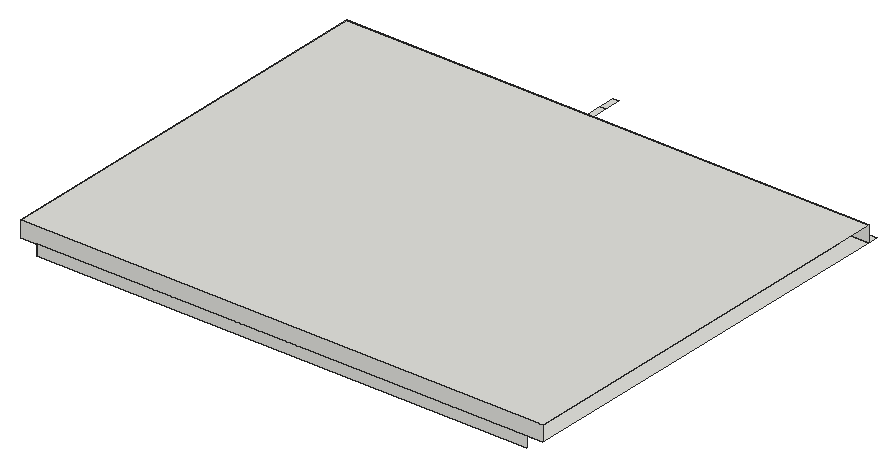
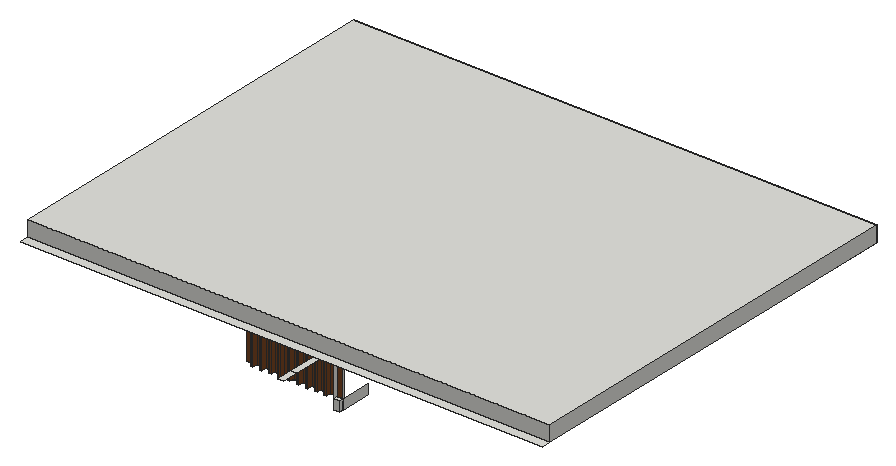
# SketchUp Ruby script. Lengths in inches.
U = 1.inch
M = Sketchup.active_model
def pt(a) = Geom::Point3d.new(a.map { |v| v * U })
def face(e, loops, mat)
  f = e.add_face(loops[0].map { |a| pt(a) })
  loops[1..].each { |l| e.add_face(l.map { |a| pt(a) }).erase! }
  f.material = f.back_material = mat if mat
  f
end
# faces: each face lists its corners as indices into pts; further lists are holes
def faces(e, pts, list, mat = nil) = list.each { |f| face(e, (f[0].is_a?(Array) ? f : [f]).map { |l| l.map { |i| pts[i] } }, mat) }
# xy, xz, yz: faces in a plane at the given z, y or x. An outline is a flat list of corners, or four numbers for a rectangle; further outlines are holes
def ring(l) = l.size == 4 ? [[l[0], l[1]], [l[2], l[1]], [l[2], l[3]], [l[0], l[3]]] : l.each_slice(2).to_a
def flat(e, list, mat, &to3) = list.each { |f| face(e, (f[0].is_a?(Array) ? f : [f]).map { |l| ring(l).map { |u, v| to3.(u, v) } }, mat) }
def xy(e, z, list, mat = nil) = flat(e, list, mat) { |x, y| [x, y, z] }
def xz(e, y, list, mat = nil) = flat(e, list, mat) { |x, z| [x, y, z] }
def yz(e, x, list, mat = nil) = flat(e, list, mat) { |y, z| [x, y, z] }
def lines(e, pts, list) = list.each { |a, b| e.add_line(pt(pts[a]), pt(pts[b])) }
# prism: a flat outline (further loops are holes) pulled along v
def prism(e, loops, v, mat = nil)
  f = face(e, loops, mat); d = Geom::Vector3d.new(v.map { |x| x * U })
  f.pushpull(f.normal.samedirection?(d) ? d.length : -d.length)
end
def box(e, o, s, mat = nil) = prism(e, [[o, [o[0] + s[0], o[1], o[2]], [o[0] + s[0], o[1] + s[1], o[2]], [o[0], o[1] + s[1], o[2]]]], [0, 0, s[2]], mat)
def at(x, y, z, deg = 0) = Geom::Transformation.translation(pt([x, y, z])) * Geom::Transformation.rotation(ORIGIN, Z_AXIS, deg.degrees)
def axes(o, x, y, z) = Geom::Transformation.new([*x, 0, *y, 0, *z, 0, *pt(o).to_a, 1])
def part(name) = M.definitions.add(name)
# library, detail: a bought-in or finely detailed component or shape, given as its bounding box
def library(name, o, s) = part(name).tap { |d| box(d.entities, o, s) }
def detail(e, o, s) = box(e.add_group.entities, o, s)
def put(e, d, t, mat = nil) = e.add_instance(d, t).tap { |i| i.material = mat if mat }
def group(e, t, mat = nil) = e.add_group.tap { |g| g.transformation = t; g.material = mat if mat }.entities
root = M.entities
M.materials.add("[Color C01]").color = [255, 229, 204]
M.materials.add("[Wood Veneer 01]").color = [120, 70, 37]
c1 = library("Avation+Styled+Ceiling+Fan_JSB",[-19.77,-29.63,-13.8125],[51.59,58.16,13.8125])
xy(root,101.64,[[84.82,147.02,87.24,148.71]])
xy(root,102.39,[[108.65,138.59,108.1,138.66,107.59,138.87,107.15,139.21,106.81,139.65,106.6,140.16,106.52,140.71,106.6,141.26,106.81,141.77,107.15,142.21,107.59,142.55,108.1,142.76,108.65,142.84,109.2,142.76,109.71,142.55,110.15,142.21,110.49,141.77,110.7,141.26,110.77,140.71,110.7,140.16,110.49,139.65,110.15,139.21,109.71,138.87,109.2,138.66]])
xy(root,105.33,[[84.82,147.02,87.24,148.71]])
xy(root,119.8125,[[87.24,147.02,89.8,148.71],[90.74,147.02,93.3,148.71],[94.24,147.02,96.8,148.71],[97.74,147.02,100.3,148.71],[101.24,147.02,103.8,148.71],
  [104.74,147.02,107.3,148.71],[108.24,147.02,110.8,148.71],[111.74,147.02,114.3,148.71],[115.24,147.02,117.8,148.71],[6.1,147.26,84.82,148.71]])
xy(root,119.8125,[[23.52,17.41,26.22,131.3],[26.64,17.41,29.35,131.3],[[29.77,17.41,32.47,131.3],[31.02,80.58,31.35,80.59,31.66,80.68,31.9375,80.85,32.16,81.08,32.32,81.37,32.4,81.6875,32.39,82.01,32.3,82.33,32.13,82.61,31.89,82.83,31.61,82.99,31.29,83.06,30.97,83.06,30.65,82.97,30.375,82.8,30.15,82.5625,29.99,82.27,29.91,81.96,29.92,81.63,30.01,81.32,30.18,81.04,30.42,80.8125,30.7,80.66]],[32.89,17.41,35.6,131.3],[36.02,17.41,38.72,131.3],
  [39.14,17.41,41.85,131.3]],"[Wood Veneer 01]")
xy(root,120.5,[[18.23,8.31,17.27,8.41,16.37,8.74,15.59,9.3,14.98,10.04,14.58,10.92,14.42,11.87,14.51,12.83,14.85,13.73,15.4,14.51,16.15,15.125,17.02,15.53,17.97,15.69,18.93,15.59,19.83,15.26,20.62,14.7,21.23,13.96,21.63,13.08,21.79,12.13,21.7,11.17,21.36,10.27,20.8,9.49,20.06,8.875,19.18,8.47],[99.22,8.5,98.3125,8.62,97.47,8.97,96.74,9.53,96.1875,10.25,95.84,11.09,95.72,12,95.84,12.91,96.1875,13.75,96.74,14.47,97.47,15.03,98.3125,15.38,99.22,15.5,100.125,15.38,100.97,15.03,101.69,14.47,102.25,13.75,102.6,12.91,102.72,12,102.6,11.09,102.25,10.25,101.69,9.53,100.97,8.97,100.125,8.62],[17.86,70.55,16.89,70.74,15.99,71.18,15.24,71.83,14.6875,72.66,14.36,73.6,14.3,74.6,14.49,75.57,14.93,76.47,15.58,77.22,16.41,77.77,17.35,78.09,18.34,78.16,19.32,77.97,20.21,77.53,20.96,76.875,21.52,76.05,21.84,75.11,21.91,74.12,21.72,73.14,21.28,72.24,20.625,71.49,19.8,70.94,18.86,70.62],[18.1,132.84,17.1,132.97,16.16,133.35,15.36,133.97,14.75,134.77,14.36,135.71,14.23,136.71,14.36,137.71,14.75,138.65,15.36,139.45,16.16,140.07,17.1,140.45,18.1,140.59,19.11,140.45,20.04,140.07,20.84,139.45,21.46,138.65,21.85,137.71,21.98,136.71,21.85,135.71,21.46,134.77,20.84,133.97,20.04,133.35,19.11,132.97],[99.22,133.4,98.36,133.51,97.5625,133.84,96.875,134.37,96.35,135.05,96.02,135.85,95.91,136.71,96.02,137.57,96.35,138.37,96.875,139.05,97.5625,139.58,98.36,139.91,99.22,140.02,100.08,139.91,100.875,139.58,101.5625,139.05,102.09,138.37,102.42,137.57,102.53,136.71,102.42,135.85,102.09,135.05,101.5625,134.37,100.875,133.84,100.08,133.51]])
xy(root,121.5,[[31.02,80.58,30.7,80.66,30.42,80.8125,30.18,81.04,30.01,81.32,29.92,81.63,29.91,81.96,29.99,82.27,30.15,82.5625,30.375,82.8,30.65,82.97,30.97,83.06,31.29,83.06,31.61,82.99,31.89,82.83,32.13,82.61,32.3,82.33,32.39,82.01,32.4,81.6875,32.32,81.37,32.16,81.08,31.9375,80.85,31.66,80.68,31.35,80.59]])
xy(root,123.25,[[26.22,17.41,26.64,131.3],[29.35,17.41,29.77,131.3],[32.47,17.41,32.89,131.3],[35.6,17.41,36.02,131.3],[38.72,17.41,39.14,131.3]])
xy(root,123.25,[[41.85,17.41,157.97,131.3]],"[Color C01]")
xy(root,123.71,[[84.82,147.02,87.07,147.26],[84.82,147.26,87.07,148.71],[84.82,148.71,87.07,154.8125],[84.82,154.8125,87.07,169.1875],[84.82,169.1875,87.07,175.3125]])
xy(root,123.75,[[0,0,0,154.8125,198.4375,154.8125,198.4375,0,192.34,0,192.34,148.71,6.1,148.71,6.1,0],[6.1,0,192.34,148.71],[0,154.8125,198.4375,158.375]])
xy(root,129.75,[[0,0,198.4375,154.8125]])
xz(root,0,[[6.1,119.8125,192.34,123.75],[0,123.75,198.4375,129.75]])
xz(root,17.41,[[26.22,119.8125,26.64,123.25],[29.35,119.8125,29.77,123.25],[32.47,119.8125,32.89,123.25],[35.6,119.8125,36.02,123.25],[38.72,119.8125,39.14,123.25],
  [41.85,119.8125,157.97,123.25]])
xz(root,83.06,[[30.97,119.8125,31.29,121.5]])
xz(root,131.3,[[26.22,119.8125,26.64,123.25],[29.35,119.8125,29.77,123.25],[32.47,119.8125,32.89,123.25],[35.6,119.8125,36.02,123.25],[38.72,119.8125,39.14,123.25]])
xz(root,131.3,[[41.85,119.8125,157.97,123.25]],"[Color C01]")
xz(root,147.02,[[84.82,101.64,87.07,105.33]])
xz(root,147.02,[[84.82,105.33,87.07,123.71],[87.24,105.33,89.8,119.8125],[90.74,105.33,93.3,119.8125],[94.24,105.33,96.8,119.8125],[97.74,105.33,100.3,119.8125],
  [101.24,105.33,103.8,119.8125],[104.74,105.33,107.3,119.8125],[108.24,105.33,110.8,119.8125],[111.74,105.33,114.3,119.8125],[115.24,105.33,117.8,119.8125],
  [118.74,105.33,121.3,119.8125]],"[Wood Veneer 01]")
xz(root,148.71,[[84.82,101.64,87.07,105.33],[87.07,101.64,87.24,105.33],[84.82,119.8125,87.07,123.71]])
xz(root,148.71,[[87.07,105.33,87.24,119.8125],[89.8,105.33,90.74,119.8125],[93.3,105.33,94.24,119.8125],[96.8,105.33,97.74,119.8125],[100.3,105.33,101.24,119.8125],
  [103.8,105.33,104.74,119.8125],[107.3,105.33,108.24,119.8125],[110.8,105.33,111.74,119.8125],[114.3,105.33,115.24,119.8125],[117.8,105.33,118.74,119.8125]],"[Wood Veneer 01]")
xz(root,154.8125,[[0,123.75,198.4375,129.75]])
yz(root,0,[[0,123.75,154.8125,129.75]])
yz(root,6.1,[[0,119.8125,148.71,123.75]])
yz(root,26.22,[[17.41,119.8125,131.3,123.25]],"[Wood Veneer 01]")
yz(root,26.64,[[17.41,119.8125,131.3,123.25]])
yz(root,29.35,[[17.41,119.8125,131.3,123.25]],"[Wood Veneer 01]")
yz(root,29.77,[[17.41,119.8125,131.3,123.25]])
yz(root,32.47,[[17.41,119.8125,131.3,123.25]],"[Wood Veneer 01]")
yz(root,32.89,[[17.41,119.8125,131.3,123.25]])
yz(root,35.6,[[17.41,119.8125,131.3,123.25]],"[Wood Veneer 01]")
yz(root,36.02,[[17.41,119.8125,131.3,123.25]],"[Wood Veneer 01]")
yz(root,38.72,[[17.41,119.8125,131.3,123.25]],"[Wood Veneer 01]")
yz(root,39.14,[[17.41,119.8125,131.3,123.25]],"[Wood Veneer 01]")
yz(root,41.85,[[17.41,119.8125,131.3,123.25]],"[Wood Veneer 01]")
yz(root,84.82,[[135.46,101.64,147.02,105.33],[147.02,101.64,147.26,105.33],[147.26,101.64,148.71,105.33],[147.02,105.33,147.26,123.71],[147.26,119.8125,148.71,123.71]])
yz(root,87.24,[[147.02,105.33,148.71,119.8125]])
yz(root,89.8,[[147.02,105.33,148.71,119.8125]],"[Wood Veneer 01]")
yz(root,90.74,[[147.02,105.33,148.71,119.8125]])
yz(root,93.3,[[147.02,105.33,148.71,119.8125]],"[Wood Veneer 01]")
yz(root,94.24,[[147.02,105.33,148.71,119.8125]])
yz(root,96.8,[[147.02,105.33,148.71,119.8125]],"[Wood Veneer 01]")
yz(root,97.74,[[147.02,105.33,148.71,119.8125]])
yz(root,100.3,[[147.02,105.33,148.71,119.8125]],"[Wood Veneer 01]")
yz(root,101.24,[[147.02,105.33,148.71,119.8125]])
yz(root,103.8,[[147.02,105.33,148.71,119.8125]],"[Wood Veneer 01]")
yz(root,104.74,[[147.02,105.33,148.71,119.8125]])
yz(root,107.3,[[147.02,105.33,148.71,119.8125]],"[Wood Veneer 01]")
yz(root,108.24,[[147.02,105.33,148.71,119.8125]])
yz(root,110.8,[[147.02,105.33,148.71,119.8125]],"[Wood Veneer 01]")
yz(root,111.74,[[147.02,105.33,148.71,119.8125]])
yz(root,114.3,[[147.02,105.33,148.71,119.8125]],"[Wood Veneer 01]")
yz(root,115.24,[[147.02,105.33,148.71,119.8125]])
yz(root,117.8,[[147.02,105.33,148.71,119.8125]],"[Wood Veneer 01]")
yz(root,118.74,[[147.02,105.33,148.71,119.8125]])
p = [[108.65,138.59,101.64],[108.1,138.66,101.64],[108.1,138.66,102.39],[108.65,138.59,102.39],[109.2,138.66,101.64],[109.2,138.66,102.39],
  [107.59,138.87,101.64],[107.59,138.87,102.39],[109.71,138.87,101.64],[109.71,138.87,102.39],[107.15,139.21,101.64],[107.15,139.21,102.39],
  [110.15,139.21,101.64],[110.15,139.21,102.39],[106.81,139.65,101.64],[106.81,139.65,102.39],[110.49,139.65,101.64],[110.49,139.65,102.39],
  [106.6,140.16,101.64],[106.6,140.16,102.39],[110.7,140.16,101.64],[110.7,140.16,102.39],[106.52,140.71,101.64],[106.52,140.71,102.39],
  [110.77,140.71,101.64],[110.77,140.71,102.39],[106.6,141.26,101.64],[106.6,141.26,102.39],[110.7,141.26,101.64],[110.7,141.26,102.39],
  [106.81,141.77,101.64],[106.81,141.77,102.39],[110.49,141.77,101.64],[110.49,141.77,102.39],[107.15,142.21,101.64],[107.15,142.21,102.39],
  [110.15,142.21,101.64],[110.15,142.21,102.39],[107.59,142.55,101.64],[107.59,142.55,102.39],[109.71,142.55,101.64],[109.71,142.55,102.39],
  [108.1,142.76,101.64],[108.1,142.76,102.39],[109.2,142.76,101.64],[109.2,142.76,102.39],[108.65,142.84,101.64],[108.65,142.84,102.39],
  [18.23,8.31,119.8125],[17.27,8.41,119.8125],[17.27,8.41,120.5],[18.23,8.31,120.5],[19.18,8.47,119.8125],[19.18,8.47,120.5],
  [16.37,8.74,119.8125],[16.37,8.74,120.5],[20.06,8.875,119.8125],[20.06,8.875,120.5],[99.22,8.5,119.8125],[98.3125,8.62,119.8125],
  [98.3125,8.62,120.5],[99.22,8.5,120.5],[100.125,8.62,119.8125],[100.125,8.62,120.5],[97.47,8.97,119.8125],[97.47,8.97,120.5],
  [100.97,8.97,119.8125],[100.97,8.97,120.5],[15.59,9.3,119.8125],[15.59,9.3,120.5],[20.8,9.49,119.8125],[20.8,9.49,120.5],
  [96.74,9.53,119.8125],[96.74,9.53,120.5],[101.69,9.53,119.8125],[101.69,9.53,120.5],[14.98,10.04,119.8125],[14.98,10.04,120.5],
  [21.36,10.27,119.8125],[21.36,10.27,120.5],[96.1875,10.25,119.8125],[96.1875,10.25,120.5],[102.25,10.25,119.8125],[102.25,10.25,120.5],
  [14.58,10.92,119.8125],[14.58,10.92,120.5],[95.84,11.09,119.8125],[95.84,11.09,120.5],[102.6,11.09,119.8125],[102.6,11.09,120.5],
  [21.7,11.17,119.8125],[21.7,11.17,120.5],[14.42,11.87,119.8125],[14.42,11.87,120.5],[95.72,12,119.8125],[95.72,12,120.5],
  [102.72,12,119.8125],[102.72,12,120.5],[21.79,12.13,119.8125],[21.79,12.13,120.5],[14.51,12.83,119.8125],[14.51,12.83,120.5],
  [95.84,12.91,119.8125],[95.84,12.91,120.5],[102.6,12.91,119.8125],[102.6,12.91,120.5],[21.63,13.08,119.8125],[21.63,13.08,120.5],
  [14.85,13.73,119.8125],[14.85,13.73,120.5],[96.1875,13.75,119.8125],[96.1875,13.75,120.5],[102.25,13.75,119.8125],[102.25,13.75,120.5],
  [21.23,13.96,119.8125],[21.23,13.96,120.5],[15.4,14.51,119.8125],[15.4,14.51,120.5],[96.74,14.47,119.8125],[96.74,14.47,120.5],
  [101.69,14.47,119.8125],[101.69,14.47,120.5],[20.62,14.7,119.8125],[20.62,14.7,120.5],[16.15,15.125,119.8125],[16.15,15.125,120.5],
  [97.47,15.03,119.8125],[97.47,15.03,120.5],[100.97,15.03,119.8125],[100.97,15.03,120.5],[19.83,15.26,119.8125],[19.83,15.26,120.5],
  [98.3125,15.38,119.8125],[98.3125,15.38,120.5],[100.125,15.38,119.8125],[100.125,15.38,120.5],[17.02,15.53,119.8125],[17.02,15.53,120.5],
  [18.93,15.59,119.8125],[18.93,15.59,120.5],[99.22,15.5,119.8125],[99.22,15.5,120.5],[17.97,15.69,119.8125],[17.97,15.69,120.5],
  [17.86,70.55,119.8125],[16.89,70.74,119.8125],[16.89,70.74,120.5],[17.86,70.55,120.5],[18.86,70.62,119.8125],[18.86,70.62,120.5],
  [19.8,70.94,119.8125],[19.8,70.94,120.5],[15.99,71.18,119.8125],[15.99,71.18,120.5],[20.625,71.49,119.8125],[20.625,71.49,120.5],
  [15.24,71.83,119.8125],[15.24,71.83,120.5],[21.28,72.24,119.8125],[21.28,72.24,120.5],[14.6875,72.66,119.8125],[14.6875,72.66,120.5],
  [21.72,73.14,119.8125],[21.72,73.14,120.5],[14.36,73.6,119.8125],[14.36,73.6,120.5],[21.91,74.12,119.8125],[21.91,74.12,120.5],
  [14.3,74.6,119.8125],[14.3,74.6,120.5],[21.84,75.11,119.8125],[21.84,75.11,120.5],[14.49,75.57,119.8125],[14.49,75.57,120.5],
  [21.52,76.05,119.8125],[21.52,76.05,120.5],[14.93,76.47,119.8125],[14.93,76.47,120.5],[20.96,76.875,119.8125],[20.96,76.875,120.5],
  [15.58,77.22,119.8125],[15.58,77.22,120.5],[20.21,77.53,119.8125],[20.21,77.53,120.5],[16.41,77.77,119.8125],[16.41,77.77,120.5],
  [19.32,77.97,119.8125],[19.32,77.97,120.5],[17.35,78.09,119.8125],[17.35,78.09,120.5],[18.34,78.16,119.8125],[18.34,78.16,120.5],
  [31.02,80.58,119.8125],[30.7,80.66,119.8125],[30.7,80.66,121.5],[31.02,80.58,121.5],[31.35,80.59,119.8125],[31.35,80.59,121.5],
  [31.66,80.68,119.8125],[31.66,80.68,121.5],[30.42,80.8125,119.8125],[30.42,80.8125,121.5],[31.9375,80.85,119.8125],[31.9375,80.85,121.5],
  [30.18,81.04,119.8125],[30.18,81.04,121.5],[32.16,81.08,119.8125],[32.16,81.08,121.5],[30.01,81.32,119.8125],[30.01,81.32,121.5],
  [32.32,81.37,119.8125],[32.32,81.37,121.5],[29.92,81.63,119.8125],[29.92,81.63,121.5],[32.4,81.6875,119.8125],[32.4,81.6875,121.5],
  [29.91,81.96,119.8125],[29.91,81.96,121.5],[32.39,82.01,119.8125],[32.39,82.01,121.5],[29.99,82.27,119.8125],[29.99,82.27,121.5],
  [32.3,82.33,119.8125],[32.3,82.33,121.5],[30.15,82.5625,119.8125],[30.15,82.5625,121.5],[32.13,82.61,119.8125],[32.13,82.61,121.5],
  [30.375,82.8,119.8125],[30.375,82.8,121.5],[31.89,82.83,119.8125],[31.89,82.83,121.5],[30.65,82.97,119.8125],[30.65,82.97,121.5],
  [31.61,82.99,119.8125],[31.61,82.99,121.5],[30.97,83.06,119.8125],[30.97,83.06,121.5],[31.29,83.06,119.8125],[31.29,83.06,121.5],
  [18.1,132.84,119.8125],[17.1,132.97,119.8125],[17.1,132.97,120.5],[18.1,132.84,120.5],[19.11,132.97,119.8125],[19.11,132.97,120.5],
  [16.16,133.35,119.8125],[16.16,133.35,120.5],[20.04,133.35,119.8125],[20.04,133.35,120.5],[15.36,133.97,119.8125],[15.36,133.97,120.5],
  [20.84,133.97,119.8125],[20.84,133.97,120.5],[99.22,133.4,119.8125],[98.36,133.51,119.8125],[98.36,133.51,120.5],[99.22,133.4,120.5],
  [100.08,133.51,119.8125],[100.08,133.51,120.5],[97.5625,133.84,119.8125],[97.5625,133.84,120.5],[100.875,133.84,119.8125],[100.875,133.84,120.5],
  [96.875,134.37,119.8125],[96.875,134.37,120.5],[101.5625,134.37,119.8125],[101.5625,134.37,120.5],[14.75,134.77,119.8125],[14.75,134.77,120.5],
  [21.46,134.77,119.8125],[21.46,134.77,120.5],[96.35,135.05,119.8125],[96.35,135.05,120.5],[102.09,135.05,119.8125],[102.09,135.05,120.5],
  [14.36,135.71,119.8125],[14.36,135.71,120.5],[21.85,135.71,119.8125],[21.85,135.71,120.5],[96.02,135.85,119.8125],[96.02,135.85,120.5],
  [102.42,135.85,119.8125],[102.42,135.85,120.5],[14.23,136.71,119.8125],[14.23,136.71,120.5],[21.98,136.71,119.8125],[21.98,136.71,120.5],
  [95.91,136.71,119.8125],[95.91,136.71,120.5],[102.53,136.71,119.8125],[102.53,136.71,120.5],[14.36,137.71,119.8125],[14.36,137.71,120.5],
  [21.85,137.71,119.8125],[21.85,137.71,120.5],[96.02,137.57,119.8125],[96.02,137.57,120.5],[102.42,137.57,119.8125],[102.42,137.57,120.5],
  [96.35,138.37,119.8125],[96.35,138.37,120.5],[102.09,138.37,119.8125],[102.09,138.37,120.5],[14.75,138.65,119.8125],[14.75,138.65,120.5],
  [21.46,138.65,119.8125],[21.46,138.65,120.5],[96.875,139.05,119.8125],[96.875,139.05,120.5],[101.5625,139.05,119.8125],[101.5625,139.05,120.5],
  [15.36,139.45,119.8125],[15.36,139.45,120.5],[20.84,139.45,119.8125],[20.84,139.45,120.5],[97.5625,139.58,119.8125],[97.5625,139.58,120.5],
  [100.875,139.58,119.8125],[100.875,139.58,120.5],[16.16,140.07,119.8125],[16.16,140.07,120.5],[20.04,140.07,119.8125],[20.04,140.07,120.5],
  [98.36,139.91,119.8125],[98.36,139.91,120.5],[100.08,139.91,119.8125],[100.08,139.91,120.5],[99.22,140.02,119.8125],[99.22,140.02,120.5],
  [17.1,140.45,119.8125],[17.1,140.45,120.5],[19.11,140.45,119.8125],[19.11,140.45,120.5],[18.1,140.59,119.8125],[18.1,140.59,120.5]]
faces(root,p,[[0,1,2,3],[4,0,3,5],[1,6,7,2],[8,4,5,9],[6,10,11,7],[12,8,9,13],[10,14,15,11],[16,12,13,17],
  [14,18,19,15],[20,16,17,21],[18,22,23,19],[24,20,21,25],[22,26,27,23],[28,24,25,29],[26,30,31,27],[32,28,29,33],
  [30,34,35,31],[36,32,33,37],[34,38,39,35],[40,36,37,41],[38,42,43,39],[44,40,41,45],[42,46,47,43],[46,44,45,47],
  [48,49,50,51],[52,48,51,53],[49,54,55,50],[56,52,53,57],[58,59,60,61],[62,58,61,63],[59,64,65,60],[66,62,63,67],
  [54,68,69,55],[70,56,57,71],[64,72,73,65],[74,66,67,75],[68,76,77,69],[78,70,71,79],[72,80,81,73],[82,74,75,83],
  [76,84,85,77],[80,86,87,81],[88,82,83,89],[90,78,79,91],[84,92,93,85],[86,94,95,87],[96,88,89,97],[98,90,91,99],
  [92,100,101,93],[94,102,103,95],[104,96,97,105],[106,98,99,107],[100,108,109,101],[102,110,111,103],[112,104,105,113],[114,106,107,115],
  [108,116,117,109],[110,118,119,111],[120,112,113,121],[122,114,115,123],[116,124,125,117],[118,126,127,119],[128,120,121,129],[130,122,123,131],
  [126,132,133,127],[134,128,129,135],[124,136,137,125],[138,130,131,139],[132,140,141,133],[140,134,135,141],[136,142,143,137],[142,138,139,143],
  [144,145,146,147],[148,144,147,149],[150,148,149,151],[145,152,153,146],[154,150,151,155],[152,156,157,153],[158,154,155,159],[156,160,161,157],
  [162,158,159,163],[160,164,165,161],[166,162,163,167],[164,168,169,165],[170,166,167,171],[168,172,173,169],[174,170,171,175],[172,176,177,173],
  [178,174,175,179],[176,180,181,177],[182,178,179,183],[180,184,185,181],[186,182,183,187],[184,188,189,185],[190,186,187,191],[188,190,191,189],
  [192,193,194,195],[196,192,195,197],[198,196,197,199],[193,200,201,194],[202,198,199,203],[200,204,205,201],[206,202,203,207],[204,208,209,205],
  [210,206,207,211],[208,212,213,209],[214,210,211,215],[212,216,217,213],[218,214,215,219],[216,220,221,217],[222,218,219,223],[220,224,225,221],
  [226,222,223,227],[224,228,229,225],[230,226,227,231],[228,232,233,229],[234,230,231,235],[232,236,237,233],[238,234,235,239],[240,241,242,243],
  [244,240,243,245],[241,246,247,242],[248,244,245,249],[246,250,251,247],[252,248,249,253],[254,255,256,257],[258,254,257,259],[255,260,261,256],
  [262,258,259,263],[260,264,265,261],[266,262,263,267],[250,268,269,251],[270,252,253,271],[264,272,273,265],[274,266,267,275],[268,276,277,269],
  [278,270,271,279],[272,280,281,273],[282,274,275,283],[276,284,285,277],[286,278,279,287],[280,288,289,281],[290,282,283,291],[284,292,293,285],
  [294,286,287,295],[288,296,297,289],[298,290,291,299],[296,300,301,297],[302,298,299,303],[292,304,305,293],[306,294,295,307],[300,308,309,301],
  [310,302,303,311],[304,312,313,305],[314,306,307,315],[308,316,317,309],[318,310,311,319],[312,320,321,313],[322,314,315,323],[316,324,325,317],
  [326,318,319,327],[324,328,329,325],[328,326,327,329],[320,330,331,321],[332,322,323,333],[330,334,335,331],[334,332,333,335]])
put(root,c1,at(97.81,75.96,123.25))
